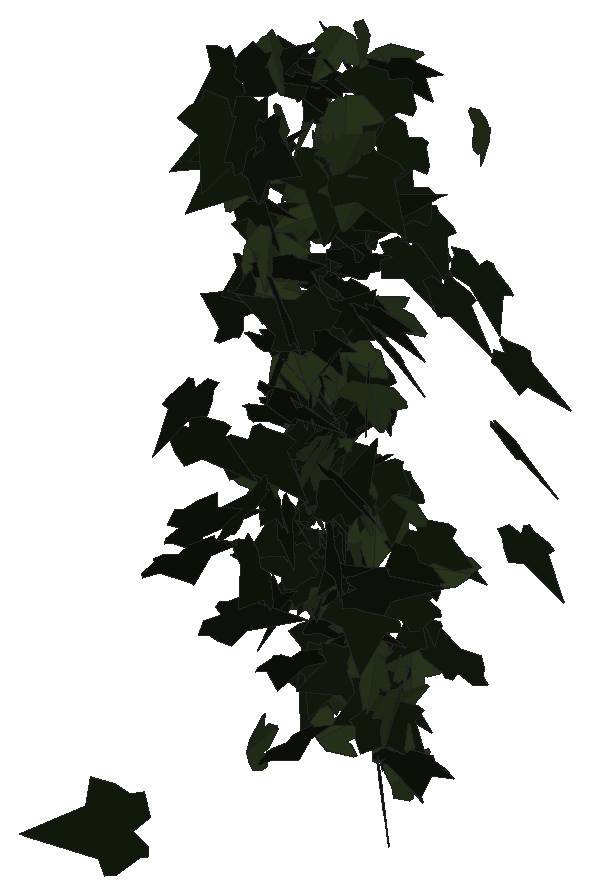
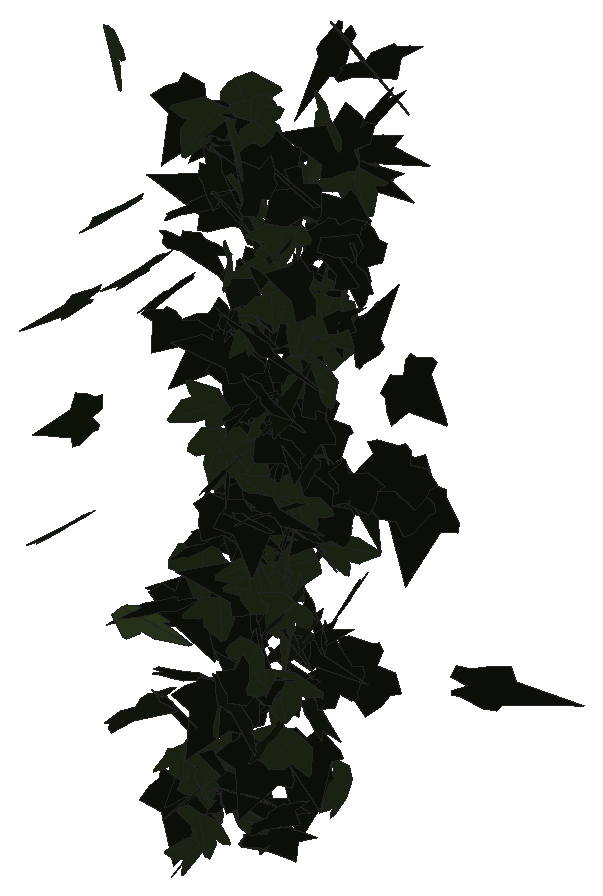
# SketchUp Ruby script. Lengths in millimetres.
U = 1.mm
M = Sketchup.active_model
def pt(a) = Geom::Point3d.new(a.map { |v| v * U })
def face(e, loops, mat)
  f = e.add_face(loops[0].map { |a| pt(a) })
  loops[1..].each { |l| e.add_face(l.map { |a| pt(a) }).erase! }
  f.material = f.back_material = mat if mat
  f
end
# faces: each face lists its corners as indices into pts; further lists are holes
def faces(e, pts, list, mat = nil) = list.each { |f| face(e, (f[0].is_a?(Array) ? f : [f]).map { |l| l.map { |i| pts[i] } }, mat) }
# xy, xz, yz: faces in a plane at the given z, y or x. An outline is a flat list of corners, or four numbers for a rectangle; further outlines are holes
def ring(l) = l.size == 4 ? [[l[0], l[1]], [l[2], l[1]], [l[2], l[3]], [l[0], l[3]]] : l.each_slice(2).to_a
def flat(e, list, mat, &to3) = list.each { |f| face(e, (f[0].is_a?(Array) ? f : [f]).map { |l| ring(l).map { |u, v| to3.(u, v) } }, mat) }
def xy(e, z, list, mat = nil) = flat(e, list, mat) { |x, y| [x, y, z] }
def xz(e, y, list, mat = nil) = flat(e, list, mat) { |x, z| [x, y, z] }
def yz(e, x, list, mat = nil) = flat(e, list, mat) { |y, z| [x, y, z] }
def lines(e, pts, list) = list.each { |a, b| e.add_line(pt(pts[a]), pt(pts[b])) }
# prism: a flat outline (further loops are holes) pulled along v
def prism(e, loops, v, mat = nil)
  f = face(e, loops, mat); d = Geom::Vector3d.new(v.map { |x| x * U })
  f.pushpull(f.normal.samedirection?(d) ? d.length : -d.length)
end
def box(e, o, s, mat = nil) = prism(e, [[o, [o[0] + s[0], o[1], o[2]], [o[0] + s[0], o[1] + s[1], o[2]], [o[0], o[1] + s[1], o[2]]]], [0, 0, s[2]], mat)
def at(x, y, z, deg = 0) = Geom::Transformation.translation(pt([x, y, z])) * Geom::Transformation.rotation(ORIGIN, Z_AXIS, deg.degrees)
def axes(o, x, y, z) = Geom::Transformation.new([*x, 0, *y, 0, *z, 0, *pt(o).to_a, 1])
def part(name) = M.definitions.add(name)
# library, detail: a bought-in or finely detailed component or shape, given as its bounding box
def library(name, o, s) = part(name).tap { |d| box(d.entities, o, s) }
def detail(e, o, s) = box(e.add_group.entities, o, s)
def put(e, d, t, mat = nil) = e.add_instance(d, t).tap { |i| i.material = mat if mat }
def group(e, t, mat = nil) = e.add_group.tap { |g| g.transformation = t; g.material = mat if mat }.entities
root = M.entities
M.materials.add("efeu1").color = [18, 25, 13]
M.materials.add("efeu2").color = [43, 57, 29]
c1 = part("ivyleaf_9")
p = [[39.1,54.8,31.7],[34.5,51.8,30.2],[-5.3,25.2,17.3],[-17.9,28.3,20.9],[-21.6,21.7,17],[-20.2,4.3,5.3],
  [-22.9,-0.3,2.5],[-17.1,-4,-0.6],[-2,-2.1,-1.2],[-0.7,-15.4,-10.1],[16.6,-22.3,-16.7],[21.1,-15.1,-12.5],
  [32.7,-10.7,-11],[46.1,-1.8,-6.6],[30.8,11.2,3.8]]
faces(c1.entities,p,[[0,1,2,3,4,5,6,7,8,9,10,11,12,13,14]],"efeu1")
c2 = part("ivyleaf_10")
p = [[0,12.8,-0.8],[-1.5,51.3,-10.9],[-4.9,51,-11.6],[-13.6,26.5,-7.3],[-13.2,15.9,-4.6],[-21.1,19.3,-7.2],
  [-29.5,16.3,-8.3],[-29.2,8.3,-6.2],[-19.7,-9.8,0.5],[-7.6,-13,4],[1,-12.2,5.8],[-0.4,51.1,-11.1],
  [-1.5,51.1,-10.9],[1,-12.4,5.9],[16.9,-12.4,3.5],[35.1,9.1,-5.1],[35,12.9,-6.1],[20.5,16.4,-4.9],
  [15.8,15,-3.8],[15.3,27.6,-7.1],[12.8,31.3,-7.8]]
faces(c2.entities,p,[[0,1,2,3,4,5,6,7,8,9,10],[11,12,0,13,14,15,16,17,18,19,20]],"efeu2")
put(root,c1,axes([654.3,876.4,1738.3],[-0.4866,-0.85576,0.34841],[-0.19614,-0.30942,-0.94404],[1.11005,-0.4298,-0.01408]))
put(root,c1,axes([631.5,650.6,2112.3],[-0.08051,-0.05628,-1.16381],[0.96456,0.85409,-0.08613],[1.04418,-0.79331,-0.01016]))
put(root,c1,axes([653.9,697.7,2574.3],[-0.24761,-0.59576,0.9813],[-0.40966,-0.92213,-0.62928],[1.33929,-0.3922,-0.01106]))
put(root,c2,axes([640,854.3,2011.7],[0.94758,0.35445,0.52156],[0.58622,0.20321,-0.85367],[-0.49822,0.91324,-0.01248]))
put(root,c2,axes([649.7,857.1,2503.5],[0.93297,0.64882,0.05094],[0.04691,0.03341,-1.00288],[-0.79261,0.76569,0.0006]))
put(root,c2,axes([681.9,724.5,2024.9],[-0.13202,0.07122,-1.061],[-1.27177,0.20355,0.11999],[0.25626,1.0469,0.04885]))
put(root,c1,axes([659.7,806.5,2232],[0.68642,0.81641,-0.26488],[-0.19927,-0.20909,-0.99139],[-1.02799,0.58567,0.0153]))
put(root,c1,axes([643.9,859.7,2007],[0.38442,-0.95114,0.23169],[0.12773,-0.20926,-1.00144],[1.18747,0.33042,0.03271]))
put(root,c1,axes([664.1,793.5,1924.6],[-0.43649,-0.56592,0.747],[-0.45966,-0.64526,-0.6693],[1.04687,-0.51928,0.01758]))
put(root,c1,axes([681,804.1,2529.9],[-0.04677,0.56451,0.88311],[-0.78284,0.68609,-0.46643],[-1.01106,-0.55734,0.32029]))
put(root,c2,axes([668.9,842.3,1898.6],[-1.25647,-0.61668,0.06954],[-0.09111,-0.05063,-0.90339],[1.17758,-0.66191,0.00431]))
put(root,c2,axes([660.1,835.2,2073.3],[-0.24142,0.93291,-0.28069],[0.03896,-0.28006,-0.95332],[-1.18791,-0.19878,0.02578]))
put(root,c1,axes([668.4,607.5,2196.5],[-0.2773,0.55334,-1.07617],[0.56734,-0.97097,-0.59746],[-1.36295,-0.51676,-0.02975]))
put(root,c1,axes([665.5,767,2338.2],[-0.63089,-0.90918,0.34186],[-0.15635,-0.32004,-1.04501],[1.17466,-0.5309,0.04451]))
put(root,c1,axes([641.8,734.5,2409.4],[-0.14452,-0.10515,-1.16065],[1.39946,0.19545,-0.13479],[0.25102,-1.15019,0.0832]))
put(root,c1,axes([653.4,767.1,2099.8],[1.21781,0.59269,0.15764],[0.18267,0.05652,-1.16057],[-0.72558,1.00899,-0.02759]))
put(root,c1,axes([635.5,724.4,2408.5],[0.70711,-0.43413,0.90897],[0.96635,-0.45147,-0.72069],[0.75923,0.97895,0.07073]))
put(root,c1,axes([674.2,761.8,2242.5],[0.05935,0.46043,1.06286],[0.05846,1.06209,-0.46229],[-1.41192,0.06333,0.02553]))
put(root,c1,axes([657.3,853.9,2476.5],[-0.22514,-0.4895,0.88906],[0.0878,-0.90767,-0.48481],[1.23507,-0.02471,0.19653]))
put(root,c2,axes([677,813.5,1967.1],[-0.93639,0.63572,0.58904],[-0.56043,0.3688,-0.99659],[-0.89659,-0.89446,0.00774]))
put(root,c2,axes([654,839.8,1821.5],[-1.06359,-0.20298,-0.65841],[0.83277,-0.11023,-0.86985],[0.11417,-1.08691,0.21117]))
put(root,c1,axes([652,728.4,2557.2],[0.14406,0.12643,1.20374],[1.22397,0.66637,-0.16841],[-0.82607,1.0094,-0.0396]))
put(root,c2,axes([665.1,806,2117.1],[1.11846,0.5159,-0.11245],[-0.13227,-0.0366,-1.05175],[-0.63045,0.92292,0.02116]))
put(root,c1,axes([672.1,782.6,1843.3],[-0.8488,0.30135,-0.64507],[0.63019,-0.40708,-0.74729],[-0.59781,-0.85701,0.12813]))
put(root,c1,axes([652.8,685.4,1854],[0.06647,0.51862,-1.1332],[0.22147,1.11888,0.5208],[1.50419,-0.18766,-0.0266]))
put(root,c1,axes([669.9,858.7,1701.9],[-0.84626,-0.80276,-0.04094],[0.0727,0.00257,-1.06004],[0.97794,-0.69486,0.04337]))
put(root,c1,axes([696.7,780.1,1906.9],[-1.08692,0.23861,0.66627],[-0.79572,0.13889,-0.92189],[-0.33509,-1.10379,0.02803]))
put(root,c1,axes([668.7,789.4,2394.3],[-0.23495,0.95956,-0.3826],[-0.33243,0.32822,0.96034],[1.21566,0.2752,0.18866]))
put(root,c1,axes([695.4,844.3,2118.5],[-0.79097,0.23991,0.70636],[-0.8237,0.20928,-0.69079],[-0.38704,-0.93567,0.0266]))
put(root,c1,axes([659.8,744.9,2457.5],[0.17136,-0.6804,-0.8475],[-0.06725,0.84899,-0.69073],[1.32422,0.13116,0.0746]))
put(root,c1,axes([673.9,841.7,2236.5],[0.62619,-0.96629,0.19404],[-0.09099,0.18007,1.094],[-1.19896,-0.51834,0.01832]))
put(root,c1,axes([656.5,719,2444.4],[0.41213,1.08296,-0.16381],[0.02519,0.1651,1.13405],[1.336,-0.33719,0.02915]))
put(root,c1,axes([676.3,687.6,2265.8],[0.15905,0.16139,1.19378],[-0.89882,-0.93933,0.20745],[1.16276,-0.74818,-0.00293]))
put(root,c1,axes([666.9,727.4,2291.4],[0.55714,-0.72078,-0.69884],[0.45314,-0.59197,0.85327],[-1.1379,-0.58865,-0.00237]))
put(root,c1,axes([689.7,675.6,2520.3],[-1.13933,-0.5715,0.59461],[-0.6017,-0.33297,-1.09462],[0.80644,-1.05585,0.02335]))
put(root,c1,axes([664.9,734.3,1839.7],[0.71311,0.70579,0.55943],[-0.43777,-0.4292,0.9164],[1.00777,-0.68586,0.00222]))
put(root,c1,axes([660,871.8,1833.2],[0.19758,-0.8234,0.56622],[0.14,-0.55449,-0.83916],[1.21108,0.19843,0.00463]))
put(root,c2,axes([679.2,704.7,2359.7],[-0.79309,0.90502,0.30084],[-0.29999,0.19273,-1.11111],[-1.1242,-0.6899,0.08426]))
put(root,c1,axes([665.2,826.2,1877.8],[0.00858,-1.02737,-0.11169],[-0.00128,0.11169,-1.02739],[1.26077,0.0071,-0.00028]))
put(root,c1,axes([700.5,835.9,2260.6],[-0.59057,0.46622,0.72834],[-0.65565,0.49175,-0.67196],[-0.82656,-0.72318,0.01262]))
put(root,c1,axes([711.3,430,1696.4],[-1.33488,-0.09018,1.0435],[-1.24531,-0.24642,-1.0916],[0.28641,-1.49177,0.11723]))
put(root,c1,axes([669.5,798.9,2533.1],[1.25559,0.29788,-0.18227],[-0.21013,-0.06049,-1.07137],[-0.37063,1.04344,-0.01008]))
put(root,c2,axes([680.7,780.8,2352.7],[-1.26579,0.09397,-0.02768],[0.03341,-0.00452,-1.04178],[-0.11475,-1.03789,0.00203]))
put(root,c1,axes([712.5,851.3,2343.3],[-1.40556,0.4433,0.41509],[-0.67126,0.21893,-0.86134],[-0.94092,-0.8184,-0.00558]))
put(root,c1,axes([661.7,796.7,1944.7],[1.02032,-0.71948,-0.22246],[-0.05472,0.28428,-1.08801],[0.91714,0.81738,0.18258]))
put(root,c2,axes([688,792.4,2004.9],[-1.11762,0.61726,0.33442],[-0.38315,0.13139,-1.1028],[-0.766,-0.96632,0.06367]))
put(root,c1,axes([663.8,779.3,1958.9],[-0.23277,-0.19871,-0.97712],[1.21285,-0.11479,-0.17078],[-0.094,-0.98894,0.21616]))
put(root,c2,axes([690.5,779.1,2459.4],[0.49721,-0.18459,0.94141],[-0.7295,0.75097,0.40611],[-0.91523,-0.69886,0.18773]))
put(root,c1,axes([678.7,763.4,2204],[-0.82418,0.23001,-0.82515],[0.94955,-0.27407,-0.71362],[-0.43646,-1.0306,0.00562]))
put(root,c1,axes([690.4,761.6,1775.9],[0.24079,0.94279,-0.38811],[-0.14523,-0.3713,-0.9625],[-1.23535,0.22742,0.03751]))
put(root,c2,axes([677.7,857.3,2008.4],[-0.1124,-0.97365,-0.06234],[0.04669,-0.06618,0.97699],[-1.18936,0.08941,0.04424]))
put(root,c1,axes([684.5,835.9,1883.7],[-0.94463,-0.75271,-0.1101],[0.12235,0.05473,-1.07943],[0.91998,-0.78016,0.03051]))
put(root,c1,axes([699.8,813.5,1971.9],[-0.88264,0.75288,0.01056],[-0.00977,0.00695,-1.04415],[-0.91855,-0.72352,0.00096]))
put(root,c1,axes([665.1,751.2,2202.7],[1.45013,0.16686,0.16905],[0.19491,0.07676,-1.1991],[-0.21444,1.19813,0.05328]))
put(root,c1,axes([684.8,842.8,1732.3],[-0.86026,-0.60463,-0.18906],[0.1946,0.10433,-0.92855],[0.74797,-0.72255,0.02413]))
put(root,c2,axes([666,751.2,2597.6],[0.78936,-0.31159,0.80284],[0.93443,-0.25085,-0.71463],[0.4803,1.00013,0.07088]))
put(root,c1,axes([698.8,673.2,2487.7],[-1.36166,-0.53671,0.2223],[-0.19755,-0.17499,-1.23545],[0.68064,-1.1245,0.08615]))
put(root,c1,axes([692.1,553.8,2007.9],[0.5478,1.35526,-0.04667],[-0.02318,-0.04287,-1.4277],[-1.65424,0.44939,0.00455]))
put(root,c2,axes([698,665.6,2526.4],[0.53554,-0.4453,-1.08934],[-0.52228,1.02258,-0.59052],[1.33739,0.57766,0.2056]))
put(root,c1,axes([706.1,777.7,1874.2],[-1.09693,0.12455,-0.45826],[-0.55153,0.07595,0.90763],[0.1774,1.00631,-0.01178]))
put(root,c1,axes([682.6,816.2,2064.5],[-0.27492,0.05875,0.9695],[-0.12799,-0.9909,0.03566],[1.17803,-0.09395,0.23013]))
put(root,c2,axes([693.7,691.9,1686.2],[0.02481,-0.00012,1.14224],[-0.55944,1.04632,0.00827],[-1.27631,-0.45864,0.01858]))
put(root,c2,axes([685,834.4,2392.9],[0.60831,0.87692,-0.15448],[-0.08316,-0.13894,-1.00872],[-1.08312,0.50316,-0.00931]))
put(root,c2,axes([668.6,797.5,2038.2],[0.369,0.29473,1.09545],[0.84223,0.85179,-0.41978],[-1.09819,0.75229,0.04613]))
put(root,c1,axes([673.9,834.4,2213.1],[-0.48689,-0.22501,-0.93669],[1.06647,0.34146,-0.45447],[0.49387,-0.9592,0.05794]))
put(root,c1,axes([694.7,804.9,2082.2],[-1.19176,-0.34915,-0.27907],[0.33153,0.06858,-1.03705],[0.43295,-1.01361,0.02596]))
put(root,c2,axes([689.6,676.1,2486],[1.14202,0.79537,-0.30071],[-0.27832,-0.19591,-1.22836],[-0.99935,0.96348,-0.00153]))
put(root,c1,axes([689.6,839.4,1792.5],[0.78331,0.8845,-0.01366],[-0.00929,-0.01135,-1.09296],[-1.07917,0.6421,-0.00051]))
put(root,c1,axes([681.9,841.1,2116],[-0.30975,-0.92079,0.03748],[-0.0082,-0.0373,-0.93506],[1.75389,-0.16279,0.00225]))
put(root,c2,axes([695.7,820.1,2227.2],[0.56401,0.70923,-0.52342],[-0.40727,-0.40614,-0.84517],[-0.99528,0.5681,0.04923]))
put(root,c1,axes([676.3,577.1,2029.2],[0.70076,0.53238,1.11167],[1.02491,0.72836,-0.78288],[-1.10036,1.01746,-0.02123]))
put(root,c2,axes([679.4,756.5,2262.5],[-0.99362,-0.01341,-0.69813],[0.85124,-0.05732,-0.81287],[-0.03311,-1.07118,0.05224]))
put(root,c2,axes([683.1,728.7,2340.3],[0.92102,0.80094,0.31522],[0.2346,0.25175,-1.1002],[-1.02356,0.77841,0.03147]))
put(root,c1,axes([674.5,867.6,2546.3],[0.30591,-0.5328,0.88166],[0.49938,-0.78117,-0.58848],[1.15331,0.47957,0.02095]))
put(root,c1,axes([717.2,771.5,2086],[-1.18263,0.71414,0.09077],[-0.08848,0.05459,-1.20403],[-0.87379,-0.97208,-0.00093]))
put(root,c1,axes([707,860.2,1766],[-0.25735,0.68411,-0.6843],[0.02591,-0.69693,-0.70328],[-1.1802,-0.16448,0.13378]))
put(root,c2,axes([685.8,831.6,2448.1],[0.04387,-0.34893,-0.93535],[0.66737,0.78983,-0.27361],[1.01883,-0.50235,0.2195]))
put(root,c1,axes([687.6,705.6,1921.6],[-0.10496,-0.78104,0.94094],[-0.09049,-0.9382,-0.78554],[1.48915,-0.11206,0.01859]))
put(root,c2,axes([681.7,817.6,2115.8],[-0.50554,-0.5741,0.82611],[0.71395,0.58916,0.70298],[-0.9983,0.71207,0.0844]))
put(root,c2,axes([678.8,841.9,2026.4],[-0.46986,-0.12615,-0.9075],[1.07526,0.21799,-0.40434],[0.30545,-0.96144,0.02739]))
put(root,c1,axes([680.2,771.5,2160.7],[1.262,-0.45759,-0.01349],[-0.01223,0.01069,-1.1311],[0.55837,1.03446,0.00572]))
put(root,c2,axes([690.5,818.2,1851.7],[-0.20126,-0.0303,1.10441],[0.64242,-0.98383,0.05166],[1.18495,0.52823,0.15957]))
put(root,c1,axes([705.5,844.4,2107.4],[0.7883,0.47342,-0.56617],[-0.61224,-0.26992,-0.79843],[-0.6602,0.8156,0.0644]))
put(root,c1,axes([709.7,830.7,2446.3],[-0.79004,0.54586,-0.58703],[0.38119,-0.52308,-0.83107],[-0.9006,-0.70025,0.1632]))
put(root,c2,axes([696.5,726.1,2313.6],[-1.2173,-0.38172,-0.40446],[0.45412,0.15888,-1.06821],[0.50412,-1.06486,-0.01439]))
put(root,c2,axes([711.1,859.4,1749.4],[0.90551,0.21167,-0.61145],[-0.73686,-0.10715,-0.77025],[-0.28318,0.95566,0.04906]))
put(root,c1,axes([693.4,855.3,1880.5],[1.1572,-0.12222,0.2382],[-0.28688,0.03888,0.95633],[-0.15615,-0.9772,0.00825]))
put(root,c2,axes([698,851.5,2041.9],[-0.22498,0.93288,-0.10467],[0.01676,-0.10398,-0.95091],[-1.14513,-0.1848,0.00665]))
put(root,c1,axes([690.7,722.9,2022],[0.02327,-0.66506,0.95638],[0.04716,-0.95562,-0.6653],[1.42038,0.04262,0.00642]))
put(root,c1,axes([710.8,781,2142.4],[0.36872,-0.19316,-1.04798],[-1.0569,0.58981,-0.35855],[0.75707,0.91746,0.00986]))
put(root,c1,axes([719.3,850.5,2097],[-1.15958,-0.05411,0.08269],[-0.09971,-0.01897,-0.95191],[0.06777,-0.95387,0.01424]))
put(root,c1,axes([677.5,744.9,2128.8],[1.09243,-0.19402,0.66311],[0.79732,-0.11428,-0.91595],[0.27344,1.10835,0.02164]))
put(root,c1,axes([688,690.7,2097.5],[-0.23776,-0.36891,-1.12579],[0.65539,0.98936,-0.4172],[1.28818,-0.57145,0.00447]))
put(root,c2,axes([685.1,715.5,2287.5],[-0.23539,-0.22256,-1.03406],[1.21991,0.30436,-0.25208],[0.42077,-1.00691,0.15236]))
put(root,c2,axes([709.3,833.9,2347.8],[0.13987,0.23421,0.95616],[-0.31288,0.93649,-0.19864],[-1.15953,-0.22444,0.16894]))
put(root,c2,axes([717.8,782.9,2376.5],[-0.24952,-0.09458,1.05284],[-0.29437,-1.03988,-0.14029],[1.25559,-0.26259,0.17634]))
put(root,c1,axes([725.7,866.1,1741.6],[-1.12799,-0.03522,0.32565],[-0.36379,-0.313,-0.88048],[0.16535,-0.92894,0.28432]))
put(root,c1,axes([689.7,774.7,2147.2],[0.88002,-0.79795,-0.19965],[0.0503,0.30029,-1.05121],[1.00225,0.68557,0.22806]))
put(root,c2,axes([690.6,838.9,1699.3],[-0.35925,0.21401,-0.87107],[0.89794,-0.46637,-0.36339],[-0.62547,-0.79245,-0.02138]))
put(root,c2,axes([699,709,2365.5],[-0.02146,-0.91105,0.71427],[0.71778,-0.62226,-0.7792],[1.21636,0.35112,0.47241]))
put(root,c2,axes([708.9,842.1,1919.3],[-1.13716,0.40462,-0.16858],[0.18611,-0.07194,-1.01612],[-0.50134,-0.94449,0.00517]))
put(root,c2,axes([699.3,761.2,2178.6],[1.16699,0.39528,0.38425],[0.34366,0.31102,-1.02118],[-0.57812,0.98281,0.16861]))
put(root,c1,axes([733.7,621.1,2047.3],[-0.49434,1.15683,0.49673],[-0.2896,0.44227,-1.22362],[-1.5084,-0.46404,0.07213]))
put(root,c1,axes([723,835,1736.4],[-0.62907,-0.42462,0.73612],[-0.52845,-0.60946,-0.65497],[0.89198,-0.66054,0.13112]))
put(root,c2,axes([727.1,776,2446.5],[0.16945,0.08286,-1.17273],[-0.50634,1.10831,0.02916],[1.34194,0.40772,0.15908]))
put(root,c1,axes([722.3,800.6,2051.5],[-1.27048,0.25838,-0.48017],[0.5705,-0.10923,-1.07294],[-0.34216,-1.14154,-0.00602]))
put(root,c2,axes([703.5,725.5,2524.1],[-0.58246,0.75238,-0.78133],[0.48456,-0.67311,-0.89087],[-1.23141,-0.62075,0.01902]))
put(root,c1,axes([729.3,840.6,2411.9],[-0.61009,0.74283,-0.45298],[0.23261,-0.41621,-0.89301],[-1.03566,-0.53107,0.06627]))
put(root,c1,axes([711,707,2338.5],[1.12076,0.69872,0.12534],[0.10862,0.08997,-1.15405],[-0.85921,0.92279,0.01761]))
put(root,c2,axes([728.9,777.2,2432.4],[-0.59007,0.76583,0.78404],[-0.58152,0.62471,-0.90425],[-1.20404,-0.67703,0.05249]))
put(root,c1,axes([708.5,790.3,2020.7],[0.60075,-0.88914,-0.4928],[-0.28693,0.43308,-1.01638],[1.20658,0.54569,0.00366]))
put(root,c1,axes([714.6,833.1,2243.8],[-0.34691,-0.98477,-0.05517],[0.01915,0.05289,-1.025],[1.20315,-0.28478,0.0004]))
put(root,c1,axes([708.2,833.2,1961.9],[-0.28267,-0.01286,-0.95951],[1.13652,-0.23981,-0.22174],[-0.28085,-0.95751,0.06842]))
put(root,c2,axes([724.3,809.3,2599.9],[0.42627,0.74419,-0.66645],[-0.37887,-0.59015,-0.82179],[-1.15838,0.46687,0.02354]))
put(root,c1,axes([716.8,771.1,2072.2],[0.59217,0.56933,0.87843],[0.45967,0.80836,-0.73211],[-1.1915,0.59482,0.15414]))
put(root,c1,axes([726.6,840.7,2345.8],[-1.10342,-0.26445,-0.32395],[0.37048,0.11534,-0.942],[0.35075,-0.95376,-0.0241]))
put(root,c1,axes([739.2,838.6,1861],[-0.55236,0.98097,0.11986],[-0.02649,0.12193,-1.07997],[-1.2054,-0.4522,-0.03119]))
put(root,c1,axes([696.7,801.4,2547.4],[0.69133,-0.21257,0.85054],[1.01453,-0.19037,-0.60161],[0.33869,1.00413,0.066]))
put(root,c2,axes([740.8,825.2,2164.1],[0.32102,0.3553,1.04017],[-0.72019,-0.85654,0.44191],[1.13119,-0.64616,-0.01384]))
put(root,c1,axes([745.7,846.7,2503.4],[-1.06324,0.50727,0.20358],[-0.21607,0.10041,-1.00839],[-0.63087,-0.88932,0.00227]))
put(root,c2,axes([728.3,771.5,2072.2],[0.17919,-1.0352,0.39436],[0.02902,-0.39477,-1.04515],[1.35118,0.14577,-0.02985]))
put(root,c1,axes([744.2,791.4,2103.9],[-0.9987,0.81752,-0.04347],[0.03753,-0.03071,-1.15692],[-0.99807,-0.81919,-0.00001]))
put(root,c1,axes([732.7,703.9,1701.6],[0.28541,1.18942,0.14616],[0.04587,0.14156,-1.21218],[-1.46129,0.23676,-0.0095]))
put(root,c1,axes([720.3,752.1,2229.5],[1.317,0.50605,-0.24222],[-0.27659,-0.08697,-1.19211],[-0.62608,1.10292,0.01713]))
put(root,c2,axes([726.9,862,2442.6],[-0.61191,0.82464,-0.3916],[-0.19598,-0.44529,-0.85315],[-1.72633,-0.24175,0.23566]))
put(root,c2,axes([716.7,809.9,2027.6],[-0.16058,-0.16156,-1.1183],[0.74276,0.93831,-0.20721],[1.16127,-0.62249,-0.0221]))
put(root,c1,axes([748.5,726.5,2255.8],[-0.04697,0.02914,1.21062],[-1.42203,-0.32935,-0.02914],[0.40063,-1.1656,0.0385]))
put(root,c2,axes([711,806.1,1661.3],[0.76723,0.00293,-0.75281],[0.91733,0.04577,0.6283],[0.04514,-0.97986,0.0271]))
put(root,c1,axes([719.1,812.9,1844.1],[0.39596,0.93277,0.0583],[-0.0827,-0.03806,0.98628],[1.1372,-0.32755,0.05143]))
put(root,c1,axes([731,598.6,2588.3],[-0.66104,-1.17495,0.20217],[-0.06747,-0.19706,-1.29348],[1.45294,-0.54372,0.03191]))
put(root,c2,axes([742.1,751.3,2055.3],[0.17345,0.02874,1.16035],[-0.64818,1.04098,0.03931],[-1.25901,-0.53197,0.13962]))
put(root,c2,axes([741.6,835.9,2595.5],[0.68599,-0.75033,-0.46469],[-0.28055,0.40741,-0.93608],[1.03955,0.60509,0.05403]))
put(root,c2,axes([739.1,833.6,2169.7],[0.72247,0.7082,-0.49333],[-0.41371,-0.35926,-0.9228],[-0.96829,0.6819,0.02619]))
put(root,c1,axes([736.8,811,2274.8],[1.14699,0.31159,-0.46753],[-0.5486,-0.12913,-0.9903],[-0.41096,1.04202,0.01708]))
put(root,c1,axes([753.2,831.8,2100.8],[-0.11239,0.81657,-0.76424],[-0.08635,-0.76955,-0.81371],[-1.36173,-0.0186,0.11468]))
put(root,c1,axes([751,780.8,2211.4],[-0.89097,0.6995,-0.61766],[0.4704,-0.48805,-1.0086],[-1.03674,-0.82259,0.07318]))
put(root,c1,axes([743.9,833.8,2336.2],[-0.28249,-0.08125,0.98555],[-0.4845,-0.91935,-0.1691],[1.10489,-0.42392,0.17783]))
put(root,c1,axes([733.5,804.6,1914.3],[0.15328,-0.2917,-1.02147],[0.84722,-0.75582,0.30125],[-0.98074,-0.69851,0.10059]))
put(root,c2,axes([747.4,836.6,1820.6],[-0.05539,-1.02151,-0.39808],[-0.02409,0.39912,-1.02192],[1.33731,-0.03512,-0.0349]))
put(root,c2,axes([744.3,793.9,2522.5],[0.58246,-0.92452,0.24382],[0.10972,-0.22789,-1.04024],[1.16131,0.48523,-0.02401]))
put(root,c1,axes([718.8,816.2,1994],[0.7406,-0.00079,0.94576],[1.1537,0.01755,-0.60697],[-0.0175,1.12369,0.01015]))
put(root,c1,axes([733.5,805.8,2219.9],[-0.56741,-0.10818,0.92864],[1.0561,-0.44162,0.3821],[0.43085,0.94003,0.28637]))
put(root,c2,axes([740,848.4,1777],[-0.9101,0.29817,-0.58635],[0.48855,-0.49749,-0.76246],[-0.63668,-0.80796,0.25308]))
put(root,c1,axes([722,830.7,1814.6],[0.68291,-0.41995,0.80627],[0.85403,-0.40498,-0.69694],[0.70759,0.89409,0.06302]))
put(root,c1,axes([778.8,581.7,2595.1],[-1.40672,0.7623,0.16219],[-0.16322,0.09174,-1.38225],[-0.93671,-1.16078,-0.00273]))
put(root,c1,axes([729.4,814,2300.2],[0.75813,0.03516,0.92551],[1.08261,0.29659,-0.60709],[-0.3236,1.0746,0.13727]))
put(root,c1,axes([752.9,841.6,1843.1],[0.87374,0.80559,0.0967],[0.01177,0.12052,-1.07547],[-0.98981,0.71256,0.07257]))
put(root,c1,axes([743.3,841.8,2152.9],[0.38914,-1.03019,-0.15265],[-0.05799,0.14508,-1.07844],[1.26924,0.32248,-0.00247]))
put(root,c1,axes([759.7,836.9,1709],[-0.34555,-0.51993,0.85137],[-0.46156,-0.76292,-0.59178],[1.12612,-0.47224,0.01869]))
put(root,c2,axes([772.5,708.6,2479.2],[1.24632,-0.0308,-0.7267],[-0.84911,0.32253,-0.99208],[0.25774,1.21148,0.24565]))
put(root,c1,axes([770.2,767.7,2045.2],[-0.95665,0.48799,-0.73843],[0.54695,-0.63164,-0.89349],[-0.93106,-0.87246,0.23385]))
put(root,c1,axes([771.7,834.6,1735.6],[-1.23147,0.32917,0.06825],[0.05203,-0.08885,1.05933],[0.40681,1.0078,0.0711]))
put(root,c2,axes([752.9,841.3,1766],[1.25719,0.1413,0.29449],[0.30094,0.30222,-1.00817],[-0.26121,1.02824,0.25585]))
put(root,c1,axes([749.9,834.8,2140.1],[-0.085,-0.08333,-1.00986],[1.11081,-0.44938,-0.02573],[-0.54252,-0.90705,0.10552]))
put(root,c2,axes([759.2,787.2,2486.3],[1.51618,-0.58142,0.10459],[0.15598,-0.06513,-0.98625],[1.11345,0.80084,-0.00427]))
put(root,c2,axes([755.8,840.5,1760.3],[1.07285,0.53234,0.32926],[0.28318,0.24999,-1.02408],[-0.7092,0.90512,0.08919]))
put(root,c1,axes([777.9,774,2050.2],[0.09739,1.17207,0.13639],[-0.05751,0.13976,-1.17344],[-1.43842,0.07377,0.05615]))
put(root,c1,axes([767,809.1,1852],[-0.59453,-0.958,-0.23688],[0.2011,0.18146,-1.07297],[1.18704,-0.51056,0.06313]))
put(root,c1,axes([790.7,741.7,2423],[-0.9294,0.93038,-0.06435],[0.05998,-0.0429,-1.20243],[-1.1362,-0.76331,-0.01084]))
put(root,c2,axes([769.3,823.8,1958.1],[0.78783,0.90057,-0.11603],[-0.09206,-0.08866,-1.10813],[-1.10395,0.65008,0.0096]))
put(root,c2,axes([760.8,844.7,2232.4],[0.50732,0.19312,0.89669],[0.78146,0.64358,-0.43565],[-0.801,0.75019,0.14291]))
put(root,c1,axes([766.1,842,1735.7],[0.79563,-0.64278,-0.53026],[-0.19371,0.56516,-0.88036],[0.99797,0.62216,0.25187]))
put(root,c1,axes([758.3,792.2,1893.9],[1.29362,0.19269,-0.25195],[0.30123,0.05044,1.0777],[0.24292,-1.0887,0.00533]))
put(root,c2,axes([786.6,796.4,2153.2],[-1.30115,-0.36356,-0.07252],[0.09151,0.0047,-1.12661],[0.44293,-1.06897,0.01971]))
put(root,c1,axes([782.1,814,2045.8],[-0.67189,-0.99492,-0.04962],[0.03404,0.04127,-1.13717],[1.21484,-0.55142,0.00442]))
put(root,c2,axes([778.4,844.1,1677],[1.28587,-0.14453,0.12272],[0.14645,-0.02787,-1.0638],[0.17905,1.06075,-0.01123]))
put(root,c1,axes([773.7,844.9,1658.9],[0.66599,-0.83394,-0.35885],[-0.2376,0.3014,-0.99672],[1.08181,0.57959,0.002]))
put(root,c1,axes([792.5,816,2521.7],[-0.83167,0.54785,-0.70155],[0.6333,-0.47315,-0.87389],[-0.88216,-0.85616,0.03403]))
put(root,c1,axes([782.8,716.7,2490.4],[-0.43856,-1.15355,-0.18065],[0.07879,0.16908,-1.20822],[1.42231,-0.36506,0.01123]))
put(root,c1,axes([793.5,574.5,2583.7],[0.44729,-0.23977,-1.36091],[-1.05479,1.05857,-0.41942],[1.31515,0.93055,0.12646]))
put(root,c2,axes([783.8,768.9,2043.3],[-0.99048,0.46034,-0.71884],[0.54698,-0.61422,-0.89972],[-0.88618,-0.89364,0.2481]))
put(root,c2,axes([788.8,791.1,1788.4],[1.26285,-0.41985,0.20856],[0.23954,-0.07078,-1.117],[0.51935,1.05355,0.00807]))
put(root,c2,axes([787.1,815.5,2593.3],[0.82707,0.69075,0.63008],[0.19386,0.68184,-0.91846],[-1.12405,0.62585,0.30521]))
put(root,c1,axes([778.4,638.7,2331.7],[0.16357,-0.60939,1.16277],[0.27323,-1.14106,-0.62384],[1.57811,0.26072,-0.01251]))
put(root,c1,axes([800.2,807,2572.3],[-0.93649,-0.84848,-0.00863],[0.00407,0.00863,-1.14418],[1.03519,-0.76762,-0.00332]))
put(root,c2,axes([795.4,736.1,2562.9],[0.56724,1.13959,-0.13152],[-0.19395,-0.07653,-1.22516],[-1.38603,0.47709,0.11762]))
put(root,c1,axes([820.7,852.5,1860.5],[-1.14983,0.08456,0.54988],[-0.66139,-0.38256,-0.87037],[0.15245,-1.0219,0.37133]))
put(root,c1,axes([816.4,686.5,2001.5],[0.43486,-0.09156,-1.2622],[-1.50524,0.26658,-0.36776],[0.34347,1.28419,-0.01365]))
put(root,c2,axes([805.6,813.9,2002.3],[-1.35814,-0.18449,0.07523],[-0.05771,-0.17006,-1.11706],[0.23612,-1.10273,0.15969]))
put(root,c1,axes([792.4,823.8,2027.6],[-0.2769,-1.06971,-0.05845],[0.16924,0.0299,-1.08585],[1.29599,-0.23246,0.12931]))
put(root,c1,axes([800.6,841.4,2479.7],[-0.59546,-0.91359,0.347],[-0.0486,-0.36895,-1.02741],[1.19128,-0.47171,0.13154]))
put(root,c2,axes([800,854.7,1768.2],[0.29231,0.99661,-0.25674],[-0.04725,-0.25469,-1.02479],[-1.25468,0.24178,-0.02122]))
put(root,c1,axes([816.1,862,1827.1],[-1.23253,0.18239,-0.18284],[0.21953,-0.03243,-1.0266],[-0.22601,-1.02617,-0.00006]))
put(root,c2,axes([807,808.9,1706.1],[1.2609,-0.12727,-0.25268],[-0.29797,0.08168,-1.04014],[0.17422,1.06083,0.04978]))
put(root,c2,axes([793.6,809.9,1715.7],[-0.19869,-0.76671,0.793],[0.42743,0.72413,0.77208],[-1.27602,0.36195,0.13515]))
put(root,c2,axes([803.5,821,1628.6],[0.27075,0.17867,-1.05559],[0.35307,1.02789,0.23482],[1.25751,-0.32707,0.16135]))
put(root,c1,axes([817.7,828.6,2423.9],[-1.28303,-0.3726,-0.10365],[0.10937,0.05726,-1.11546],[0.45898,-1.0552,-0.02393]))
put(root,c1,axes([807.7,712.4,2039.6],[-0.33817,-0.46797,1.12575],[1.07187,0.72371,0.51717],[-1.03117,0.90575,0.16841]))
put(root,c1,axes([806.9,806.6,2598.1],[1.21116,0.58947,-0.08514],[-0.09181,-0.04003,-1.15456],[-0.72079,0.99559,0.00399]))
put(root,c1,axes([802,775.2,2274.9],[1.41704,0.09295,-0.04965],[-0.06053,-0.00236,-1.16522],[-0.11342,1.16257,0.00161]))
put(root,c1,axes([806.2,791.6,1726.9],[-0.07342,-0.55867,-0.99023],[0.1183,0.98548,-0.56188],[1.38203,-0.11404,-0.00451]))
put(root,c1,axes([804.2,850.1,2328.6],[-0.47423,-0.56207,-0.84526],[0.77474,0.57147,-0.67204],[0.96613,-0.73416,0.12401]))
put(root,c1,axes([843.6,809.3,1937.7],[0.32006,0.32968,-1.02575],[-1.14809,-0.44397,-0.38337],[-0.64007,0.96119,0.17475]))
put(root,c1,axes([815.5,684.7,2100.5],[1.52314,-0.12602,-0.34378],[-0.40778,0.10643,-1.25288],[0.18236,1.29056,0.06975]))
put(root,c1,axes([814.9,859.5,2370.5],[0.27197,-1.02597,-0.19339],[0.04641,0.2056,-1.0469],[1.27288,0.21172,0.07949]))
put(root,c2,axes([839,711,2486.5],[-0.72919,-1.01434,0.36921],[-0.13978,-0.36003,-1.17461],[1.30949,-0.60327,0.08021]))
put(root,c2,axes([838.9,696.6,2552.5],[-0.43016,-1.17768,0.2315],[-0.12575,-0.21068,-1.22875],[1.45886,-0.36541,-0.03765]))
put(root,c1,axes([832.8,799.8,1676.7],[1.07839,0.61677,-0.46369],[-0.47551,-0.25166,-1.07773],[-0.81248,0.96592,0.0153]))
put(root,c2,axes([830,781.8,1761.7],[0.27245,-1.12722,0.31047],[0.25378,-0.27274,-1.13984],[1.40366,0.2681,0.14582]))
put(root,c1,axes([816.1,772.5,1655.9],[-0.03233,-0.00046,-1.20975],[1.39522,-0.3946,-0.0249],[-0.48129,-1.14389,0.00907]))
put(root,c1,axes([813,741.4,1921.3],[0.3985,0.66507,-0.97805],[0.42876,0.91426,0.73906],[1.37779,-0.47687,0.05289]))
put(root,c1,axes([819.8,845.4,1951.9],[0.628,-0.56215,-0.65112],[0.08424,0.70755,-0.58844],[1.635,0.17946,0.28041]))
put(root,c1,axes([817.8,736.5,2431.2],[0.41667,-0.01169,1.21299],[1.43872,0.29849,-0.32917],[-0.34679,1.2243,0.09184]))
put(root,c2,axes([873.1,848.8,1915.7],[-0.05157,1.23527,0.10042],[-1.5114,-0.04494,0.03131],[0.04249,-0.09925,1.2356]))
put(root,c1,axes([826.5,759.2,2260],[0.81816,-0.8364,0.47804],[0.41632,-0.33846,-1.0709],[1.09912,0.7508,0.04979]))
put(root,c1,axes([877.7,841.1,1791.4],[-0.22288,1.18347,0.00538],[-1.44328,-0.18277,0.03272],[0.04045,-0.00033,1.19704]))
put(root,c1,axes([836.2,709.5,2512.8],[0.12294,-0.97999,-0.75342],[0.35013,0.75382,-0.94212],[1.46688,-0.09779,0.28802]))
put(root,c1,axes([903.6,788.9,2337.8],[0.71086,-0.88306,-0.24384],[-0.12346,0.23718,-0.95828],[1.73915,0.37778,0.03164]))
put(root,c1,axes([958.2,783,2387.3],[0.12487,-0.98315,0.16665],[0.0258,-0.16611,-0.98533],[1.89764,0.06695,0.00243]))
put(root,c1,axes([954.2,832,2141],[1.26318,-0.68917,-0.03715],[-0.07261,0.01483,-0.95665],[1.31152,0.66459,-0.01718]))
put(root,c2,axes([987.1,752.8,2595.4],[0.84313,-0.76352,-0.53721],[-0.23434,0.54164,-0.87136],[1.76125,0.43757,0.14123]))
put(root,c1,axes([972.3,847.1,2000.1],[0.51891,-0.86727,-0.22469],[-0.04249,0.22822,-0.90796],[1.70455,0.26971,0.04577]))
put(root,c1,axes([987.5,800.6,2271],[1.14112,-0.60968,-0.48435],[-0.27019,0.51547,-0.82459],[1.45711,0.57305,0.22641]))
